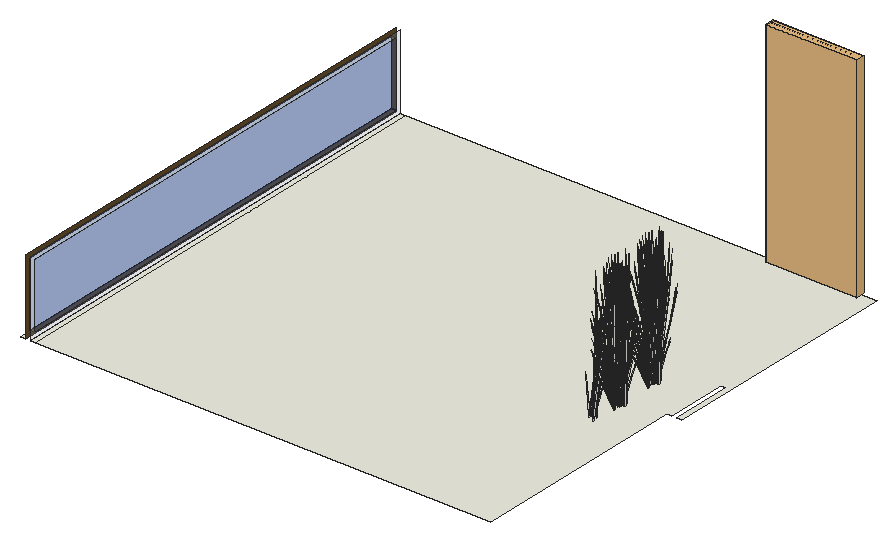
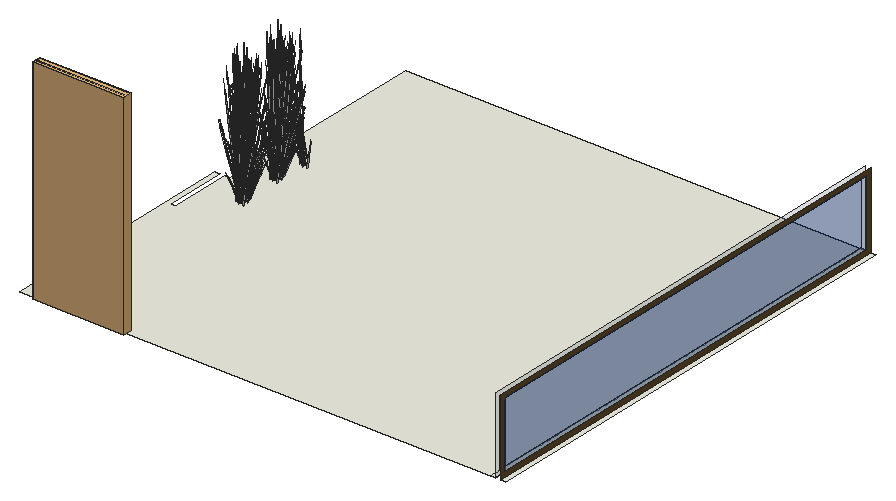
# SketchUp Ruby script. Lengths in inches.
U = 1.inch
M = Sketchup.active_model
def pt(a) = Geom::Point3d.new(a.map { |v| v * U })
def face(e, loops, mat)
  f = e.add_face(loops[0].map { |a| pt(a) })
  loops[1..].each { |l| e.add_face(l.map { |a| pt(a) }).erase! }
  f.material = f.back_material = mat if mat
  f
end
# faces: each face lists its corners as indices into pts; further lists are holes
def faces(e, pts, list, mat = nil) = list.each { |f| face(e, (f[0].is_a?(Array) ? f : [f]).map { |l| l.map { |i| pts[i] } }, mat) }
# xy, xz, yz: faces in a plane at the given z, y or x. An outline is a flat list of corners, or four numbers for a rectangle; further outlines are holes
def ring(l) = l.size == 4 ? [[l[0], l[1]], [l[2], l[1]], [l[2], l[3]], [l[0], l[3]]] : l.each_slice(2).to_a
def flat(e, list, mat, &to3) = list.each { |f| face(e, (f[0].is_a?(Array) ? f : [f]).map { |l| ring(l).map { |u, v| to3.(u, v) } }, mat) }
def xy(e, z, list, mat = nil) = flat(e, list, mat) { |x, y| [x, y, z] }
def xz(e, y, list, mat = nil) = flat(e, list, mat) { |x, z| [x, y, z] }
def yz(e, x, list, mat = nil) = flat(e, list, mat) { |y, z| [x, y, z] }
def lines(e, pts, list) = list.each { |a, b| e.add_line(pt(pts[a]), pt(pts[b])) }
# prism: a flat outline (further loops are holes) pulled along v
def prism(e, loops, v, mat = nil)
  f = face(e, loops, mat); d = Geom::Vector3d.new(v.map { |x| x * U })
  f.pushpull(f.normal.samedirection?(d) ? d.length : -d.length)
end
def box(e, o, s, mat = nil) = prism(e, [[o, [o[0] + s[0], o[1], o[2]], [o[0] + s[0], o[1] + s[1], o[2]], [o[0], o[1] + s[1], o[2]]]], [0, 0, s[2]], mat)
def at(x, y, z, deg = 0) = Geom::Transformation.translation(pt([x, y, z])) * Geom::Transformation.rotation(ORIGIN, Z_AXIS, deg.degrees)
def axes(o, x, y, z) = Geom::Transformation.new([*x, 0, *y, 0, *z, 0, *pt(o).to_a, 1])
def part(name) = M.definitions.add(name)
# library, detail: a bought-in or finely detailed component or shape, given as its bounding box
def library(name, o, s) = part(name).tap { |d| box(d.entities, o, s) }
def detail(e, o, s) = box(e.add_group.entities, o, s)
def put(e, d, t, mat = nil) = e.add_instance(d, t).tap { |i| i.material = mat if mat }
def group(e, t, mat = nil) = e.add_group.tap { |g| g.transformation = t; g.material = mat if mat }.entities
root = M.entities
M.materials.add("D01_Frost_White").color = [238, 238, 227]
M.materials.add("Glass_Basic_01").color = [161, 173, 186]
M.materials["Glass_Basic_01"].alpha = 0.25
M.materials.add("Glass_Sky Reflection_01").color = [0, 46, 142]
M.materials["Glass_Sky Reflection_01"].alpha = 0.25
M.materials.add("LightPink_Translucent").color = [144, 107, 117]
M.materials["LightPink_Translucent"].alpha = 0.75
M.materials.add("Wood_Veneer_15_1K").color = [103, 79, 44]
c1 = part("blade")
p = [[2.15,0.21,22],[0,0.17,0],[0.09,0.45,0],[2.18,0.31,22],[2.29,0.31,22],[0.38,0.45,0],
  [2.48,0.24,33],[2.49,0.24,33],[2.48,0.22,33]]
faces(c1.entities,p,[[0,1,2,3],[4,5,2,3],[6,3,4,7],[8,0,3,6]])
c2 = part("seeds")
p = [[0.3,-0.1,1.38],[-0.01,-0.03,1.59],[-0.01,-0.03,0.03],[0.14,-0.07,-0.07],[0.29,-0.03,3],[0.15,0.01,3.11]]
faces(c2.entities,p,[[0,1,2,3],[1,0,4,5]],"LightPink_Translucent")
c3 = part("blade with seeds")
put(c3.entities,c1,at(0,0,0))
put(c3.entities,c2,axes([2.4,0.25,30.99],[1.5799,-0.05474,1.17369],[-0.12525,1.92788,0.29478],[-0.07173,-0.02425,1.56792]))
c4 = library("porta+4",[0.2,-5.42,1.33],[46.55,4.72,83.21])
xy(root,147,[[124,178,126,361],[128,178,130,361],[130,178,310,178,310,265,312,265,312,289,314,289,314,265,316,265,316,361,130,361]],"D01_Frost_White")
xy(root,149,[[126,180,128,359]],"Glass_Basic_01")
xz(root,359,[[126,149,128,175]],"Glass_Basic_01")
xz(root,361,[[[274,147,310,231],[277,150,307,228]]],"Wood_Veneer_15_1K")
yz(root,126,[[180,149,359,175]],"Glass_Sky Reflection_01")
yz(root,126,[[[178,147,361,177],[180,149,359,175]]],"Wood_Veneer_15_1K")
yz(root,128,[[[178,147,361,177],[180,149,359,175]]],"Glass_Basic_01")
yz(root,128,[[180,149,359,175]],"Glass_Sky Reflection_01")
put(root,c3,axes([296.94,246.52,149],[0.25622,0.47263,0],[-0.42866,0.26357,-0.43598],[-0.09763,0.06003,1.38303]))
put(root,c3,axes([296.72,244.65,149.4],[-0.01119,-0.44408,1.19347],[0.50665,0.11511,0.50532],[-0.11983,0.243,1.12654]))
put(root,c3,axes([296.85,245.13,148.77],[0.15027,0.43184,-0.5847],[-0.43285,0.15553,-0.15346],[0.01661,0.14623,1.29063]))
put(root,c3,axes([293.9,246.62,148.26],[0.05497,0.04712,1.48974],[0.09321,0.43661,-0.22758],[-0.12183,0.0931,0.25375]))
put(root,c3,axes([294.9,247.34,149.34],[-0.01061,-0.28045,0.97034],[0.26501,0.20003,0.71294],[-0.05212,0.13367,0.21373]))
put(root,c3,axes([295.6,246.67,148.26],[0.06632,-0.02567,1.48974],[0.39894,0.14126,-0.22758],[0.01167,0.15921,0.25375]))
put(root,c3,axes([295,246.25,151.23],[0.29336,0.31691,-0.47917],[-0.3099,0.27755,-0.37115],[-0.04464,0.16102,0.91684]))
put(root,c3,axes([294.68,246.73,149.38],[0.37228,-0.08352,0.05498],[0.08559,0.3365,-0.7291],[-0.0236,0.17034,0.65354]))
put(root,c3,axes([295.87,246.56,150.95],[0.40284,0.11824,-0.43168],[-0.13808,0.40538,-0.33437],[0.03694,0.16321,0.82598]))
put(root,c3,axes([294.91,246.11,151.51],[-0.01066,0.43628,-0.66621],[-0.44902,-0.0293,0.0804],[-0.04739,0.18483,0.94242]))
put(root,c3,axes([295.72,246.48,151.21],[0.19559,0.38351,-0.60019],[-0.40262,0.21373,0.07243],[0.04574,0.1853,0.84903]))
put(root,c3,axes([294.59,247.09,149.1875],[0.12932,-0.07441,1.20808],[0.31929,0.22435,-0.25981],[-0.09503,0.19413,0.51652]))
put(root,c3,axes([294.76,246.72,149.84],[0.009,-0.24349,1.30391],[0.40497,0.12861,0.18019],[-0.03509,0.2595,0.61571]))
put(root,c3,axes([297.69,255.92,151.21],[-0.19559,-0.38351,-0.60019],[0.40262,-0.21373,0.07243],[-0.04574,-0.1853,0.84903]))
put(root,c3,axes([296.42,255.41,149.1875],[-0.02482,0.15429,1.20808],[-0.36278,0.12916,-0.25981],[-0.0848,-0.19943,0.51652]))
put(root,c3,axes([297.36,255.07,148.26],[-0.06874,0.01699,1.48974],[-0.38012,-0.19128,-0.22758],[0.00638,-0.15955,0.25375]))
put(root,c3,axes([297.73,255.59,150.82],[0.12355,-0.36271,-0.29918],[0.36044,0.10579,0.38624],[-0.03305,-0.14603,0.73904]))
put(root,c3,axes([297.55,255.84,150.95],[-0.40284,-0.11824,-0.43168],[0.13808,-0.40538,-0.33437],[-0.03694,-0.16321,0.82598]))
put(root,c3,axes([297.8,254.83,149.34],[0.05257,0.27504,0.97034],[-0.29163,-0.15233,0.71294],[0.03138,-0.14083,0.21373]))
put(root,c3,axes([296.3,255.16,149.34],[0.21377,0.16416,0.97034],[-0.31132,0.09868,0.71294],[-0.06661,-0.12616,0.21373]))
put(root,c3,axes([296.8125,256.03,151.21],[-0.34944,-0.22798,-0.60019],[0.24834,-0.39949,0.07243],[-0.1266,-0.13612,0.84903]))
put(root,c3,axes([296.69,255.73,150.82],[-0.06329,-0.37991,-0.29918],[0.36182,-0.10032,0.38624],[-0.09718,-0.10887,0.73904]))
put(root,c3,axes([296.13,255.65,148.26],[-0.0397,0.06213,1.48974],[-0.40116,0.13396,-0.22758],[-0.09691,-0.12186,0.25375]))
put(root,c3,axes([296.79,257.36,148.77],[-0.1683,-0.48366,-0.58997],[0.48479,-0.17419,-0.15484],[-0.0186,-0.16378,1.30225]))
put(root,c3,axes([296.65,256.04,150.95],[-0.40438,0.11212,-0.43168],[-0.07074,-0.4246,-0.33437],[-0.10862,-0.12168,0.82598]))
put(root,c3,axes([296.72,255.97,149],[-0.25622,-0.47263,0],[0.42866,-0.26357,-0.43598],[0.09763,-0.06003,1.38303]))
put(root,c3,axes([297.29,255.4,148.8],[-0.28319,0.27058,-0.03288],[-0.25948,-0.29635,-0.1491],[-0.01827,-0.08397,0.4918]))
put(root,c3,axes([297.65,258.61,149.81],[0.35414,0.19019,1.27785],[-0.34693,0.40974,0.50532],[-0.1554,-0.24285,1.07126]))
put(root,c3,axes([295.8,257.29,148.7],[0,-0.47166,-0.41945],[0.45849,0,0],[0,-0.10742,1.33059]))
put(root,c3,axes([297.04,257.49,148.87],[0.19883,-0.425,-0.37796],[0.41314,0.20454,0.1819],[0,-0.09797,1.2135]))
put(root,c3,axes([295.85,256.39,150.82],[-0.23317,-0.29531,-0.29918],[0.26625,-0.27955,0.38624],[-0.13527,-0.04253,0.73904]))
put(root,c3,axes([295.99,257.3,148.71],[0.28606,-0.29428,-0.2617],[0.28606,0.29428,0.2617],[0,-0.09479,1.17405]))
put(root,c3,axes([295.88,255.89,148.8],[-0.11822,0.38513,-0.03288],[-0.36385,-0.11847,-0.1491],[-0.05524,-0.06299,0.4918]))
put(root,c3,axes([297,257.84,149.25],[-0.46151,-0.22505,-0.2458],[0.22222,-0.475,-0.42242],[-0.0145,-0.11662,1.34921]))
put(root,c3,axes([295.68,257.65,149],[-0.51243,0,0],[0,-0.52715,-0.43598],[0,-0.12006,1.38303]))
put(root,c3,axes([295.77,256.71,149.1875],[0.08001,0.13132,1.20808],[-0.18437,0.35694,-0.25981],[-0.18931,-0.08532,0.51652]))
put(root,c3,axes([296.1,256.59,151.21],[-0.40965,-0.01136,-0.60019],[0.02751,-0.47821,0.07243],[-0.17355,-0.05047,0.84903]))
put(root,c3,axes([296.08,257.51,148.97],[-0.38118,0.39654,0.25983],[-0.38142,-0.39237,-0.30828],[-0.01331,-0.11261,1.39295]))
put(root,c3,axes([297.29,257.7,149.06],[0.46174,0.2286,0.2033],[-0.22222,0.475,0.42242],[0,-0.1095,1.35626]))
put(root,c3,axes([297.11,258.34,149.06],[0.10862,-0.55889,-0.19793],[0.515,0.09742,0.43313],[-0.08999,-0.07718,1.32161]))
put(root,c3,axes([295.96,256.6875,150.95],[-0.29757,0.31243,-0.43168],[-0.2606,-0.33005,-0.33437],[-0.15119,-0.04754,0.82598]))
put(root,c3,axes([295.29,257.1,149.34],[0.26163,-0.03375,0.97034],[-0.16596,0.29737,0.71294],[-0.12929,-0.04461,0.21373]))
put(root,c3,axes([297.14,257.38,149.3],[-0.44501,0.02912,0.37796],[-0.04024,-0.48332,-0.1819],[0.07967,-0.04899,1.2135]))
put(root,c3,axes([295.99,257.73,149.09],[0,0.47166,0.41945],[-0.45849,0,0],[0,-0.10742,1.33059]))
put(root,c3,axes([297.08,258.11,148.87],[-0.24618,-0.39589,-0.37796],[0.37289,-0.27878,0.1819],[-0.07967,-0.04899,1.2135]))
put(root,c3,axes([297.125,257.55,148.99],[0.17817,0.52741,0.38653],[-0.50909,0.1834,0.15168],[0.00622,-0.09691,1.34202]))
put(root,c3,axes([297.04,257.97,149.3],[-0.19883,0.425,0.37796],[-0.41314,-0.20454,-0.1819],[0,-0.09797,1.2135]))
put(root,c3,axes([297.77,257.6,148.86],[0,-0.54574,0],[0.51243,0,0],[0,0,1.51605]))
put(root,c3,axes([296.85,258.26,148.74],[-0.42629,-0.07733,-0.52676],[0.08996,-0.47699,-0.13825],[-0.12722,-0.0578,1.16273]))
put(root,c3,axes([297.9,258.02,148.94],[-0.38118,-0.40596,-0.0518],[0.38142,-0.40621,0],[-0.01331,-0.01418,1.48322]))
put(root,c3,axes([296.93,256.55,149.09],[-0.11838,0.46875,0.14904],[-0.43321,-0.13265,0.29641],[0.07483,-0.00228,1.35512]))
put(root,c3,axes([297.17,258.07,148.99],[0.51796,0.09937,0.38653],[-0.10541,0.56124,0.15168],[-0.07569,-0.05419,1.34202]))
put(root,c3,axes([295.48,257.59,148.26],[0.01039,0.07433,1.48974],[-0.20952,0.38819,-0.22758],[-0.14882,-0.01957,0.25375]))
put(root,c3,axes([296.4,258.99,148.71],[-0.09626,-0.41098,-0.2617],[0.38233,-0.1167,0.2617],[-0.07708,-0.04739,1.17405]))
put(root,c3,axes([296.89,258.97,149.09],[0.44036,-0.12519,0.14904],[0.10874,0.46588,0.29641],[-0.03927,-0.06788,1.35512]))
put(root,c3,axes([296.3,259.17,148.7],[-0.38354,-0.23583,-0.41945],[0.22925,-0.42288,0],[-0.08735,-0.05371,1.33059]))
put(root,c3,axes([295.44,257.42,150.82],[-0.34057,-0.13158,-0.29918],[0.09933,-0.38387,0.38624],[-0.13712,0.0352,0.73904]))
put(root,c3,axes([297.34,258.33,149.25],[-0.41376,0.31314,-0.2458],[-0.27514,-0.44246,-0.42242],[-0.10209,-0.04493,1.34921]))
put(root,c3,axes([298.25,256.57,149.09],[-0.44036,0.12519,0.14904],[-0.10874,-0.46588,0.29641],[0.03927,0.06788,1.35512]))
put(root,c3,axes([297.55,258.86,148.86],[-0.13371,-0.40664,0],[0.38182,-0.1424,0],[0,0,1.30413]))
put(root,c3,axes([297.3,258.47,149.21],[-0.07906,0.42093,0.12232],[-0.38625,-0.07307,-0.3493],[-0.07029,-0.04322,1.07074]))
put(root,c3,axes([298.2,258.99,149.09],[0.11838,-0.46875,0.14904],[0.43321,0.13265,0.29641],[-0.07483,0.00228,1.35512]))
put(root,c3,axes([296.48,257.36,149.82],[0.11649,-0.06823,1.49584],[0.04017,0.47639,0.11706],[-0.25231,0.06321,0.53462]))
put(root,c3,axes([298.88,257.79,149.09],[-0.32198,-0.34356,0.14904],[0.32447,-0.33323,0.29641],[-0.03556,0.07016,1.35512]))
put(root,c3,axes([297.46,259.04,148.86],[-0.41314,-0.21175,0],[0.19883,-0.43999,0],[0,0,1.37455]))
put(root,c3,axes([297.8,258.48,149.08],[-0.40016,-0.37963,-0.21282],[0.33672,-0.42629,0.46574],[-0.10776,0.04441,1.42109]))
put(root,c3,axes([296.75,259.2,149.09],[0.38354,0.23583,0.41945],[-0.22925,0.42288,0],[-0.08735,-0.05371,1.33059]))
put(root,c3,axes([298.03,257.8125,148.9375],[0,0.54548,-0.04762],[-0.51243,0,0],[0,0.01714,1.5153]))
put(root,c3,axes([295.68,257.62,150.95],[-0.11102,0.42903,-0.43168],[-0.38064,-0.14706,-0.33437],[-0.15325,0.03934,0.82598]))
put(root,c3,axes([296.53,259.45,149],[-0.25622,0.47263,0],[-0.42866,-0.26357,-0.43598],[-0.09763,-0.06003,1.38303]))
put(root,c3,axes([298,258.16,149.3],[0.44501,-0.02912,0.37796],[0.04024,0.48332,-0.1819],[-0.07967,0.04899,1.2135]))
put(root,c3,axes([297.6,258.4,148.87],[-0.44501,0.02912,-0.37796],[-0.04024,-0.48332,0.1819],[-0.07967,0.04899,1.2135]))
put(root,c3,axes([298.09,259.52,148.85],[-0.25302,-0.47428,-0.04344],[0.42866,-0.26357,0.43598],[-0.10563,0.04516,1.38235]))
put(root,c3,axes([298,258.37,149.21],[0.30276,0.28338,0.12232],[-0.25254,0.31972,-0.3493],[-0.07029,0.04322,1.07074]))
put(root,c3,axes([298.33,259.24,149.09],[0.38354,-0.23583,0.41945],[0.22925,0.42288,0],[-0.08735,0.05371,1.33059]))
put(root,c3,axes([297.78,258.87,148.9375],[0.17817,0.54185,-0.05079],[-0.50909,0.18987,0],[0.00622,0.01892,1.45452]))
put(root,c3,axes([297.98,259.46,148.71],[-0.38233,-0.1167,-0.2617],[0.09626,-0.41098,0.2617],[-0.07708,0.04739,1.17405]))
put(root,c3,axes([295.22,258.62,149.1875],[0.14242,0.03872,1.20808],[0.09179,0.39548,-0.25981],[-0.19345,0.07403,0.51652]))
put(root,c3,axes([299.25,258.16,148.86],[-0.51218,-0.00377,-0.04204],[0,-0.52715,0.42192],[-0.0161,0.12,1.33776]))
put(root,c3,axes([294.92,259.45,149.34],[0.17079,-0.21377,0.97034],[0.06739,0.33841,0.71294],[-0.12342,0.0606,0.21373]))
put(root,c3,axes([297.91,258.26,149.25],[0.04775,0.53819,-0.2458],[-0.49736,0.03254,-0.42242],[-0.08758,0.07169,1.34921]))
put(root,c3,axes([298.09,258.05,148.87],[-0.19883,0.425,-0.37796],[-0.41314,-0.20454,0.1819],[0,0.09797,1.2135]))
put(root,c3,axes([295.57,258.53,150.82],[-0.35672,0.06741,-0.29918],[-0.09419,-0.38534,0.38624],[-0.10222,0.1035,0.73904]))
put(root,c3,axes([297.61,258.68,148.74],[-0.27603,0.35451,-0.52676],[-0.34289,-0.32147,-0.13825],[-0.11061,0.08844,1.16273]))
put(root,c3,axes([298.1,259.27,148.97],[0.51304,0.1533,0.25983],[-0.12835,0.54797,-0.30828],[-0.08491,0.06858,1.39295]))
put(root,c3,axes([298.07,259.64,148.7],[-0.38354,0.23583,-0.41945],[-0.22925,-0.42288,0],[-0.08735,0.05371,1.33059]))
put(root,c3,axes([295.86,258.57,150.95],[0.10528,0.43067,-0.43168],[-0.39868,0.07534,-0.33437],[-0.11425,0.11568,0.82598]))
put(root,c3,axes([298.42,259.57,149],[0.25622,0.47263,0],[-0.42866,0.26357,-0.43598],[-0.09763,0.06003,1.38303]))
put(root,c3,axes([298.2,257.7,149.4],[-0.01119,-0.44408,1.19347],[0.50665,0.11511,0.50532],[-0.11983,0.243,1.12654]))
put(root,c3,axes([295.37,259.67,148.26],[0.05497,0.04712,1.48974],[0.09321,0.43661,-0.22758],[-0.12183,0.0931,0.25375]))
put(root,c3,axes([296.19,259.42,150.82],[-0.27728,0.24833,-0.29918],[-0.26248,-0.28355,0.38624],[-0.03994,0.14407,0.73904]))
put(root,c3,axes([296.37,260.38,149.34],[-0.01061,-0.28045,0.97034],[0.26501,0.20003,0.71294],[-0.05212,0.13367,0.21373]))
put(root,c3,axes([297.07,259.71,148.26],[0.06632,-0.02567,1.48974],[0.39894,0.14126,-0.22758],[0.01167,0.15921,0.25375]))
put(root,c3,axes([296.47,259.3,151.23],[0.29336,0.31691,-0.47917],[-0.3099,0.27755,-0.37115],[-0.04464,0.16102,0.91684]))
put(root,c3,axes([296.15,259.78,149.38],[0.37228,-0.08352,0.05498],[0.08559,0.3365,-0.7291],[-0.0236,0.17034,0.65354]))
put(root,c3,axes([297.16,259.86,150.82],[-0.12355,0.36271,-0.29918],[-0.36044,-0.10579,0.38624],[0.03305,0.14603,0.73904]))
put(root,c3,axes([296.38,259.16,151.51],[-0.01066,0.43628,-0.66621],[-0.44902,-0.0293,0.0804],[-0.04739,0.18483,0.94242]))
put(root,c3,axes([297.19,259.53,151.21],[0.19559,0.38351,-0.60019],[-0.40262,0.21373,0.07243],[0.04574,0.1853,0.84903]))
put(root,c3,axes([296.0625,260.13,149.1875],[0.12932,-0.07441,1.20808],[0.31929,0.22435,-0.25981],[-0.09503,0.19413,0.51652]))
put(root,c3,axes([296.23,259.77,149.84],[0.009,-0.24349,1.30391],[0.40497,0.12861,0.18019],[-0.03509,0.2595,0.61571]))
put(root,c3,axes([296.98,273.53,151.21],[-0.19559,-0.38351,-0.60019],[0.40262,-0.21373,0.07243],[-0.04574,-0.1853,0.84903]))
put(root,c3,axes([295.71,273.01,149.1875],[-0.02482,0.15429,1.20808],[-0.36278,0.12916,-0.25981],[-0.0848,-0.19943,0.51652]))
put(root,c3,axes([296.64,272.67,148.26],[-0.06874,0.01699,1.48974],[-0.38012,-0.19128,-0.22758],[0.00638,-0.15955,0.25375]))
put(root,c3,axes([296.83,273.45,150.95],[-0.40284,-0.11824,-0.43168],[0.13808,-0.40538,-0.33437],[-0.03694,-0.16321,0.82598]))
put(root,c3,axes([297.08,272.43,149.34],[0.05257,0.27504,0.97034],[-0.29163,-0.15233,0.71294],[0.03138,-0.14083,0.21373]))
put(root,c3,axes([297.7,273.76,150.95],[-0.29336,-0.31691,-0.43168],[0.3099,-0.27755,-0.33437],[0.04464,-0.16102,0.82598]))
put(root,c3,axes([295.58,272.76,149.34],[0.21377,0.16416,0.97034],[-0.31132,0.09868,0.71294],[-0.06661,-0.12616,0.21373]))
put(root,c3,axes([296.1,273.63,151.21],[-0.34944,-0.22798,-0.60019],[0.24834,-0.39949,0.07243],[-0.1266,-0.13612,0.84903]))
put(root,c3,axes([295.41,273.26,148.26],[-0.0397,0.06213,1.48974],[-0.40116,0.13396,-0.22758],[-0.09691,-0.12186,0.25375]))
put(root,c3,axes([296.07,274.97,148.77],[-0.1683,-0.48366,-0.58997],[0.48479,-0.17419,-0.15484],[-0.0186,-0.16378,1.30225]))
put(root,c3,axes([295.93,273.65,150.95],[-0.40438,0.11212,-0.43168],[-0.07074,-0.4246,-0.33437],[-0.10862,-0.12168,0.82598]))
put(root,c3,axes([296.01,273.58,149],[-0.25622,-0.47263,0],[0.42866,-0.26357,-0.43598],[0.09763,-0.06003,1.38303]))
put(root,c3,axes([296.57,273.01,148.8],[-0.28319,0.27058,-0.03288],[-0.25948,-0.29635,-0.1491],[-0.01827,-0.08397,0.4918]))
put(root,c3,axes([296.93,276.21,149.81],[0.35414,0.19019,1.27785],[-0.34693,0.40974,0.50532],[-0.1554,-0.24285,1.07126]))
put(root,c3,axes([295.08,274.9,148.7],[0,-0.47166,-0.41945],[0.45849,0,0],[0,-0.10742,1.33059]))
put(root,c3,axes([296.33,275.09,148.87],[0.19883,-0.425,-0.37796],[0.41314,0.20454,0.1819],[0,-0.09797,1.2135]))
put(root,c3,axes([296.51,274.88,149.25],[-0.04775,-0.53819,-0.2458],[0.49736,-0.03254,-0.42242],[0.08758,-0.07169,1.34921]))
put(root,c3,axes([295.28,274.91,148.71],[0.28606,-0.29428,-0.2617],[0.28606,0.29428,0.2617],[0,-0.09479,1.17405]))
put(root,c3,axes([295.16,273.5,148.8],[-0.11822,0.38513,-0.03288],[-0.36385,-0.11847,-0.1491],[-0.05524,-0.06299,0.4918]))
put(root,c3,axes([296.28,275.44,149.25],[-0.46151,-0.22505,-0.2458],[0.22222,-0.475,-0.42242],[-0.0145,-0.11662,1.34921]))
put(root,c3,axes([294.97,275.26,149],[-0.51243,0,0],[0,-0.52715,-0.43598],[0,-0.12006,1.38303]))
put(root,c3,axes([295.05,274.31,149.1875],[0.08001,0.13132,1.20808],[-0.18437,0.35694,-0.25981],[-0.18931,-0.08532,0.51652]))
put(root,c3,axes([296.45,273.6875,148.71],[0.38233,0.1167,-0.2617],[-0.09626,0.41098,0.2617],[0.07708,-0.04739,1.17405]))
put(root,c3,axes([295.39,274.2,151.21],[-0.40965,-0.01136,-0.60019],[0.02751,-0.47821,0.07243],[-0.17355,-0.05047,0.84903]))
put(root,c3,axes([295.36,275.12,148.97],[-0.38118,0.39654,0.25983],[-0.38142,-0.39237,-0.30828],[-0.01331,-0.11261,1.39295]))
put(root,c3,axes([296.58,275.3,149.06],[0.46174,0.2286,0.2033],[-0.22222,0.475,0.42242],[0,-0.1095,1.35626]))
put(root,c3,axes([296.4,275.94,149.06],[0.10862,-0.55889,-0.19793],[0.515,0.09742,0.43313],[-0.08999,-0.07718,1.32161]))
put(root,c3,axes([295.25,274.29,150.95],[-0.29757,0.31243,-0.43168],[-0.2606,-0.33005,-0.33437],[-0.15119,-0.04754,0.82598]))
put(root,c3,axes([294.58,274.71,149.34],[0.26163,-0.03375,0.97034],[-0.16596,0.29737,0.71294],[-0.12929,-0.04461,0.21373]))
put(root,c3,axes([296.43,274.98,149.3],[-0.44501,0.02912,0.37796],[-0.04024,-0.48332,-0.1819],[0.07967,-0.04899,1.2135]))
put(root,c3,axes([295.28,275.34,149.09],[0,0.47166,0.41945],[-0.45849,0,0],[0,-0.10742,1.33059]))
put(root,c3,axes([296.36,275.72,148.87],[-0.24618,-0.39589,-0.37796],[0.37289,-0.27878,0.1819],[-0.07967,-0.04899,1.2135]))
put(root,c3,axes([296.41,275.16,148.99],[0.17817,0.52741,0.38653],[-0.50909,0.1834,0.15168],[0.00622,-0.09691,1.34202]))
put(root,c3,axes([296.32,275.57,149.3],[-0.19883,0.425,0.37796],[-0.41314,-0.20454,-0.1819],[0,-0.09797,1.2135]))
put(root,c3,axes([297.05,275.2,148.86],[0,-0.54574,0],[0.51243,0,0],[0,0,1.51605]))
put(root,c3,axes([296.14,275.87,148.74],[-0.42629,-0.07733,-0.52676],[0.08996,-0.47699,-0.13825],[-0.12722,-0.0578,1.16273]))
put(root,c3,axes([296.81,274.86,148.99],[-0.33979,0.42804,0.38653],[-0.40368,-0.37784,0.15168],[0.08192,-0.04272,1.34202]))
put(root,c3,axes([297.18,275.625,148.94],[-0.38118,-0.40596,-0.0518],[0.38142,-0.40621,0],[-0.01331,-0.01418,1.48322]))
put(root,c3,axes([296.22,274.15,149.09],[-0.11838,0.46875,0.14904],[-0.43321,-0.13265,0.29641],[0.07483,-0.00228,1.35512]))
put(root,c3,axes([296.46,275.68,148.99],[0.51796,0.09937,0.38653],[-0.10541,0.56124,0.15168],[-0.07569,-0.05419,1.34202]))
put(root,c3,axes([294.77,275.2,148.26],[0.01039,0.07433,1.48974],[-0.20952,0.38819,-0.22758],[-0.14882,-0.01957,0.25375]))
put(root,c3,axes([296.96,274.79,149.3],[-0.24618,-0.39589,0.37796],[0.37289,-0.27878,-0.1819],[0.07967,0.04899,1.2135]))
put(root,c3,axes([295.6875,276.6,148.71],[-0.09626,-0.41098,-0.2617],[0.38233,-0.1167,0.2617],[-0.07708,-0.04739,1.17405]))
put(root,c3,axes([296.18,276.57,149.09],[0.44036,-0.12519,0.14904],[0.10874,0.46588,0.29641],[-0.03927,-0.06788,1.35512]))
put(root,c3,axes([295.58,276.77,148.7],[-0.38354,-0.23583,-0.41945],[0.22925,-0.42288,0],[-0.08735,-0.05371,1.33059]))
put(root,c3,axes([297.4,275.32,148.86],[0.45849,0,0],[0,0.4883,0],[0,0,1.50718]))
put(root,c3,axes([296.625,275.9375,149.25],[-0.41376,0.31314,-0.2458],[-0.27514,-0.44246,-0.42242],[-0.10209,-0.04493,1.34921]))
put(root,c3,axes([297.53,274.18,149.09],[-0.44036,0.12519,0.14904],[-0.10874,-0.46588,0.29641],[0.03927,0.06788,1.35512]))
put(root,c3,axes([297.25,275.08,149.01],[-0.51796,-0.09937,0.41563],[0.10541,-0.56124,0.1631],[0.07569,0.05419,1.44303]))
put(root,c3,axes([296.84,276.46,148.86],[-0.13371,-0.40664,0],[0.38182,-0.1424,0],[0,0,1.30413]))
put(root,c3,axes([296.58,276.08,149.21],[-0.07906,0.42093,0.12232],[-0.38625,-0.07307,-0.3493],[-0.07029,-0.04322,1.07074]))
put(root,c3,axes([297.49,276.6,149.09],[0.11838,-0.46875,0.14904],[0.43321,0.13265,0.29641],[-0.07483,0.00228,1.35512]))
put(root,c3,axes([297.39,275.53,148.87],[0.28606,0.30466,0],[-0.28606,0.30466,0],[0,0,1.42996]))
put(root,c3,axes([295.76,274.96,149.82],[0.11649,-0.06823,1.49584],[0.04017,0.47639,0.11706],[-0.25231,0.06321,0.53462]))
put(root,c3,axes([298.16,275.4,149.09],[-0.32198,-0.34356,0.14904],[0.32447,-0.33323,0.29641],[-0.03556,0.07016,1.35512]))
put(root,c3,axes([296.75,276.65,148.86],[-0.41314,-0.21175,0],[0.19883,-0.43999,0],[0,0,1.37455]))
put(root,c3,axes([297.09,276.08,149.08],[-0.40016,-0.37963,-0.21282],[0.33672,-0.42629,0.46574],[-0.10776,0.04441,1.42109]))
put(root,c3,axes([296.03,276.81,149.09],[0.38354,0.23583,0.41945],[-0.22925,0.42288,0],[-0.08735,-0.05371,1.33059]))
put(root,c3,axes([297.39,275.18,149.3],[0.19883,-0.425,0.37796],[0.41314,0.20454,-0.1819],[0,0.09797,1.2135]))
put(root,c3,axes([297.31,275.42,148.9375],[0,0.54548,-0.04762],[-0.51243,0,0],[0,0.01714,1.5153]))
put(root,c3,axes([294.96,275.22,150.95],[-0.11102,0.42903,-0.43168],[-0.38064,-0.14706,-0.33437],[-0.15325,0.03934,0.82598]))
put(root,c3,axes([295.8125,277.06,149],[-0.25622,0.47263,0],[-0.42866,-0.26357,-0.43598],[-0.09763,-0.06003,1.38303]))
put(root,c3,axes([297.28,275.77,149.3],[0.44501,-0.02912,0.37796],[0.04024,0.48332,-0.1819],[-0.07967,0.04899,1.2135]))
put(root,c3,axes([297.56,275.27,149.21],[0.38182,-0.13755,0.12232],[0.13371,0.39278,-0.3493],[0,0.08644,1.07074]))
put(root,c3,axes([296.89,276,148.87],[-0.44501,0.02912,-0.37796],[-0.04024,-0.48332,0.1819],[-0.07967,0.04899,1.2135]))
put(root,c3,axes([297.21,276.65,148.86],[0.41314,0.21175,0],[-0.19883,0.43999,0],[0,0,1.47801]))
put(root,c3,axes([297.38,277.12,148.85],[-0.25302,-0.47428,-0.04344],[0.42866,-0.26357,0.43598],[-0.10563,0.04516,1.38235]))
put(root,c3,axes([297.29,275.98,149.21],[0.30276,0.28338,0.12232],[-0.25254,0.31972,-0.3493],[-0.07029,0.04322,1.07074]))
put(root,c3,axes([297.61,276.85,149.09],[0.38354,-0.23583,0.41945],[0.22925,0.42288,0],[-0.08735,0.05371,1.33059]))
put(root,c3,axes([297.07,276.48,148.9375],[0.17817,0.54185,-0.05079],[-0.50909,0.18987,0],[0.00622,0.01892,1.45452]))
put(root,c3,axes([297.26,277.0625,148.71],[-0.38233,-0.1167,-0.2617],[0.09626,-0.41098,0.2617],[-0.07708,0.04739,1.17405]))
put(root,c3,axes([294.5,276.23,149.1875],[0.14242,0.03872,1.20808],[0.09179,0.39548,-0.25981],[-0.19345,0.07403,0.51652]))
put(root,c3,axes([298.54,275.77,148.86],[-0.51218,-0.00377,-0.04204],[0,-0.52715,0.42192],[-0.0161,0.12,1.33776]))
put(root,c3,axes([297.43,275.31,149.25],[0.46151,0.22505,-0.2458],[-0.22222,0.475,-0.42242],[0.0145,0.11662,1.34921]))
put(root,c3,axes([294.21,277.06,149.34],[0.17079,-0.21377,0.97034],[0.06739,0.33841,0.71294],[-0.12342,0.0606,0.21373]))
put(root,c3,axes([298.43,275.84,148.71],[-0.28606,0.29428,-0.2617],[-0.28606,-0.29428,0.2617],[0,0.09479,1.17405]))
put(root,c3,axes([297.2,275.87,149.25],[0.04775,0.53819,-0.2458],[-0.49736,0.03254,-0.42242],[-0.08758,0.07169,1.34921]))
put(root,c3,axes([297.38,275.66,148.87],[-0.19883,0.425,-0.37796],[-0.41314,-0.20454,0.1819],[0,0.09797,1.2135]))
put(root,c3,axes([296.9,276.28,148.74],[-0.27603,0.35451,-0.52676],[-0.34289,-0.32147,-0.13825],[-0.11061,0.08844,1.16273]))
put(root,c3,axes([297.39,276.88,148.97],[0.51304,0.1533,0.25983],[-0.12835,0.54797,-0.30828],[-0.08491,0.06858,1.39295]))
put(root,c3,axes([297.35,277.25,148.7],[-0.38354,0.23583,-0.41945],[-0.22925,-0.42288,0],[-0.08735,0.05371,1.33059]))
put(root,c3,axes([295.15,276.18,150.95],[0.10528,0.43067,-0.43168],[-0.39868,0.07534,-0.33437],[-0.11425,0.11568,0.82598]))
put(root,c3,axes([297.7,277.18,149],[0.25622,0.47263,0],[-0.42866,0.26357,-0.43598],[-0.09763,0.06003,1.38303]))
put(root,c3,axes([297.48,275.3,149.4],[-0.01119,-0.44408,1.19347],[0.50665,0.11511,0.50532],[-0.11983,0.243,1.12654]))
put(root,c3,axes([297.61,275.79,148.77],[0.15027,0.43184,-0.5847],[-0.43285,0.15553,-0.15346],[0.01661,0.14623,1.29063]))
put(root,c3,axes([294.66,277.28,148.26],[0.05497,0.04712,1.48974],[0.09321,0.43661,-0.22758],[-0.12183,0.0931,0.25375]))
put(root,c3,axes([295.66,277.99,149.34],[-0.01061,-0.28045,0.97034],[0.26501,0.20003,0.71294],[-0.05212,0.13367,0.21373]))
put(root,c3,axes([296.35,277.32,148.26],[0.06632,-0.02567,1.48974],[0.39894,0.14126,-0.22758],[0.01167,0.15921,0.25375]))
put(root,c3,axes([295.76,276.91,151.23],[0.29336,0.31691,-0.47917],[-0.3099,0.27755,-0.37115],[-0.04464,0.16102,0.91684]))
put(root,c3,axes([295.4375,277.38,149.38],[0.37228,-0.08352,0.05498],[0.08559,0.3365,-0.7291],[-0.0236,0.17034,0.65354]))
put(root,c3,axes([296.625,277.21,150.95],[0.40284,0.11824,-0.43168],[-0.13808,0.40538,-0.33437],[0.03694,0.16321,0.82598]))
put(root,c3,axes([295.66,276.76,151.51],[-0.01066,0.43628,-0.66621],[-0.44902,-0.0293,0.0804],[-0.04739,0.18483,0.94242]))
put(root,c3,axes([296.48,277.14,151.21],[0.19559,0.38351,-0.60019],[-0.40262,0.21373,0.07243],[0.04574,0.1853,0.84903]))
put(root,c3,axes([295.35,277.74,149.1875],[0.12932,-0.07441,1.20808],[0.31929,0.22435,-0.25981],[-0.09503,0.19413,0.51652]))
put(root,c3,axes([295.51,277.38,149.84],[0.009,-0.24349,1.30391],[0.40497,0.12861,0.18019],[-0.03509,0.2595,0.61571]))
put(root,c4,axes([273.84,363.0625,145.65],[0.77339,0,0],[0,0.75842,0],[0,0,1.0096]),"D01_Frost_White")
